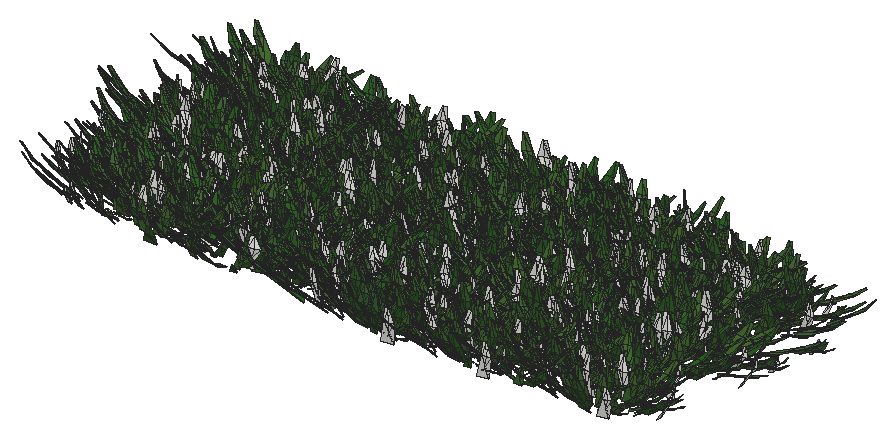
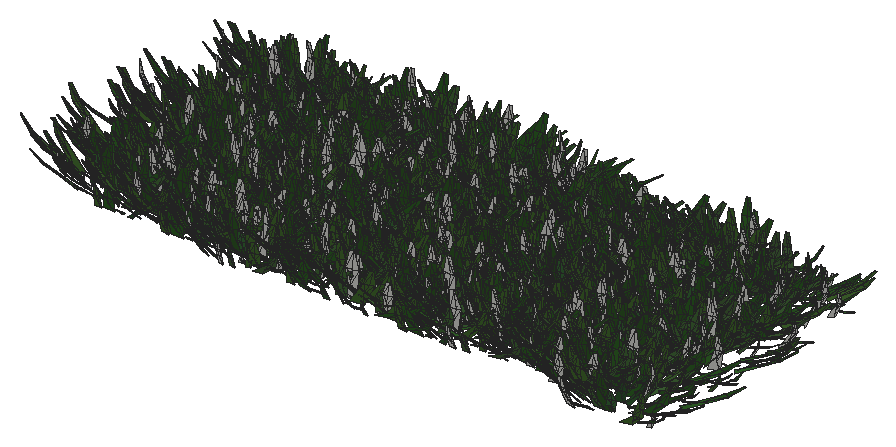
# SketchUp Ruby script. Lengths in inches.
U = 1.inch
M = Sketchup.active_model
def pt(a) = Geom::Point3d.new(a.map { |v| v * U })
def face(e, loops, mat)
  f = e.add_face(loops[0].map { |a| pt(a) })
  loops[1..].each { |l| e.add_face(l.map { |a| pt(a) }).erase! }
  f.material = f.back_material = mat if mat
  f
end
# faces: each face lists its corners as indices into pts; further lists are holes
def faces(e, pts, list, mat = nil) = list.each { |f| face(e, (f[0].is_a?(Array) ? f : [f]).map { |l| l.map { |i| pts[i] } }, mat) }
# xy, xz, yz: faces in a plane at the given z, y or x. An outline is a flat list of corners, or four numbers for a rectangle; further outlines are holes
def ring(l) = l.size == 4 ? [[l[0], l[1]], [l[2], l[1]], [l[2], l[3]], [l[0], l[3]]] : l.each_slice(2).to_a
def flat(e, list, mat, &to3) = list.each { |f| face(e, (f[0].is_a?(Array) ? f : [f]).map { |l| ring(l).map { |u, v| to3.(u, v) } }, mat) }
def xy(e, z, list, mat = nil) = flat(e, list, mat) { |x, y| [x, y, z] }
def xz(e, y, list, mat = nil) = flat(e, list, mat) { |x, z| [x, y, z] }
def yz(e, x, list, mat = nil) = flat(e, list, mat) { |y, z| [x, y, z] }
def lines(e, pts, list) = list.each { |a, b| e.add_line(pt(pts[a]), pt(pts[b])) }
# prism: a flat outline (further loops are holes) pulled along v
def prism(e, loops, v, mat = nil)
  f = face(e, loops, mat); d = Geom::Vector3d.new(v.map { |x| x * U })
  f.pushpull(f.normal.samedirection?(d) ? d.length : -d.length)
end
def box(e, o, s, mat = nil) = prism(e, [[o, [o[0] + s[0], o[1], o[2]], [o[0] + s[0], o[1] + s[1], o[2]], [o[0], o[1] + s[1], o[2]]]], [0, 0, s[2]], mat)
def at(x, y, z, deg = 0) = Geom::Transformation.translation(pt([x, y, z])) * Geom::Transformation.rotation(ORIGIN, Z_AXIS, deg.degrees)
def axes(o, x, y, z) = Geom::Transformation.new([*x, 0, *y, 0, *z, 0, *pt(o).to_a, 1])
def part(name) = M.definitions.add(name)
# library, detail: a bought-in or finely detailed component or shape, given as its bounding box
def library(name, o, s) = part(name).tap { |d| box(d.entities, o, s) }
def detail(e, o, s) = box(e.add_group.entities, o, s)
def put(e, d, t, mat = nil) = e.add_instance(d, t).tap { |i| i.material = mat if mat }
def group(e, t, mat = nil) = e.add_group.tap { |g| g.transformation = t; g.material = mat if mat }.entities
root = M.entities
M.materials.add("Material82").color = [68, 110, 58]
M.materials.add("Material83").color = [48, 90, 38]
M.materials.add("Material84").color = [68, 110, 48]
M.materials.add("Material85").color = [48, 90, 48]
M.materials.add("Material86").color = [58, 110, 58]
M.materials.add("Material87").color = [58, 90, 38]
M.materials.add("Material88").color = [68, 100, 58]
M.materials.add("Material89").color = [48, 100, 38]
c1 = part("grass00")
p = [[-0.6875,0.15,0],[-0.56,0.08,5.52],[-0.04,0.03,2.76],[0.48,-0.02,0],[0.35,-0.02,5.52],[-0.1,-0.14,5.52],
  [-0.12,0.65,8.37],[-0.42,0.65,8.37]]
faces(c1.entities,p,[[0,1,2,3],[3,2,4],[1,5,2],[5,4,2],[1,6,5],[4,5,6],[7,6,1]])
c2 = part("Group16\#1")
put(c2.entities,c1,axes([1.44,-0.61,-0.01],[0.05352,0.12609,0],[-0.10704,0.04543,0.07239],[0.06664,-0.02828,0.11628]),"Material85")
put(c2.entities,c1,axes([0.76,-0.15,-0.01],[0.04676,0.24062,0],[-0.23162,0.04501,0.06642],[0.0652,-0.01267,0.23595]),"Material82")
put(c2.entities,c1,axes([0.79,0.01,-0.01],[-0.00606,0.34651,0],[-0.34381,-0.00602,0.0432],[0.04319,0.00076,0.34386]))
put(c2.entities,c1,axes([1,0.23,-0.01],[-0.07192,0.31144,0],[-0.28722,-0.06632,0.1236],[0.12043,0.02781,0.29478]),"Material84")
put(c2.entities,c1,axes([1.66,0.77,-0.01],[-0.13828,0.29651,0],[-0.21551,-0.1005,0.22471],[0.20365,0.09498,0.23779]),"Material89")
put(c2.entities,c1,axes([0.6875,0.52,-0.01],[-0.18126,0.24051,0],[-0.22746,-0.17142,0.09788],[0.07817,0.05891,0.28481]),"Material84")
put(c2.entities,c1,axes([0.68,0.78,-0.01],[-0.215,0.18688,0],[-0.12385,-0.14248,0.21334],[0.13995,0.16101,0.18878]),"Material82")
put(c2.entities,c1,axes([0.56,1,-0.01],[-0.13756,0.07624,0],[-0.06159,-0.11112,0.0927],[0.04494,0.08108,0.12705]),"Material84")
put(c2.entities,c1,axes([0.2,0.64,-0.01],[-0.23729,0.07254,0],[-0.05711,-0.18681,0.153],[0.04473,0.14632,0.19535]),"Material89")
put(c2.entities,c1,axes([0.0625,0.72,-0.01],[-0.28874,0.02525,0],[-0.02179,-0.24916,0.14647],[0.01276,0.14591,0.25012]),"Material82")
put(c2.entities,c1,axes([-0.08,0.62,-0.01],[-0.34089,-0.04187,0],[0.03255,-0.26504,0.216],[-0.02633,0.21439,0.26703]),"Material89")
put(c2.entities,c1,axes([-0.34,0.98,-0.01],[-0.14314,-0.0493,0],[0.04397,-0.12769,0.06843],[-0.02228,0.0647,0.13505]),"Material89")
put(c2.entities,c1,axes([-0.87,1.45,-0.01],[-0.23488,-0.14114,0],[0.13761,-0.22901,0.06087],[-0.03135,0.05217,0.26717]))
put(c2.entities,c1,axes([-0.72,0.77,-0.01],[-0.14208,-0.13251,0],[0.07209,-0.0773,0.16301],[-0.11118,0.11922,0.1057]),"Material89")
put(c2.entities,c1,axes([-0.62,0.43,-0.01],[-0.14845,-0.21203,0],[0.18654,-0.13061,0.12304],[-0.10079,0.07057,0.22772]),"Material82")
put(c2.entities,c1,axes([-0.68,0.29,-0.01],[-0.13639,-0.32136,0],[0.31723,-0.13464,0.05579],[-0.05136,0.0218,0.34462]),"Material83")
put(c2.entities,c1,axes([-0.64,0.125,-0.01],[-0.0458,-0.23569,0],[0.22124,-0.043,0.08276],[-0.08124,0.01579,0.22538]),"Material86")
put(c2.entities,c1,axes([-1.6,-0.03,-0.01],[0.00576,-0.32897,0],[0.27526,0.00482,0.18018],[-0.18015,-0.00315,0.2753]),"Material84")
put(c2.entities,c1,axes([-1.36,-0.31,-0.01],[0.05718,-0.24765,0],[0.18172,0.04196,0.17267],[-0.16825,-0.03885,0.1865]),"Material89")
put(c2.entities,c1,axes([-1.54,-0.72,-0.01],[0.06537,-0.14017,0],[0.13555,0.06321,0.03939],[-0.0357,-0.01665,0.14956]))
put(c2.entities,c1,axes([-1.19,-0.9,-0.01],[0.09597,-0.12735,0],[0.11214,0.08451,0.07557],[-0.06035,-0.04548,0.14042]),"Material88")
put(c2.entities,c1,axes([-0.47,-0.54,-0.01],[0.11588,-0.10072,0],[0.0618,0.0711,0.12124],[-0.07953,-0.0915,0.0942]))
put(c2.entities,c1,axes([-0.47,-0.84,-0.01],[0.11927,-0.0661,0],[0.06603,0.11913,0.00646],[-0.00313,-0.00565,0.13621]),"Material84")
put(c2.entities,c1,axes([-0.38,-1.24,-0.01],[0.28037,-0.08571,0],[0.0618,0.20215,0.20315],[-0.05939,-0.19428,0.21139]),"Material88")
put(c2.entities,c1,axes([-0.06,-0.66,-0.01],[0.22719,-0.01987,0],[0.01247,0.14255,0.17758],[-0.01547,-0.17691,0.1431]),"Material87")
put(c2.entities,c1,axes([0.11,-0.89,-0.01],[0.14882,0.01828,0],[-0.01058,0.08611,0.12229],[0.01491,-0.12138,0.08676]),"Material85")
put(c2.entities,c1,axes([0.25,-0.72,-0.01],[0.20481,0.07053,0],[-0.06206,0.18022,0.10291],[0.03351,-0.0973,0.1906]),"Material85")
put(c2.entities,c1,axes([0.85,-1.42,-0.01],[0.16481,0.09904,0],[-0.09472,0.15762,0.05616],[0.02893,-0.04814,0.18389]),"Material84")
put(c2.entities,c1,axes([1.01,-1.09,-0.01],[0.21858,0.20385,0],[-0.17495,0.1876,0.15339],[0.10462,-0.11218,0.25652]),"Material89")
put(c2.entities,c1,axes([1.01,-0.71,-0.01],[0.08733,0.12473,0],[-0.06445,0.04512,0.13037],[0.1068,-0.07477,0.07867]),"Material85")
c3 = part("Group15\#1")
put(c3.entities,c2,at(0,0,0))
c4 = part("3darcstudiotree_grass00\#1")
put(c4.entities,c3,at(0,0,0))
put(root,c4,axes([1732.89,309.77,-34.17],[-4.54038,0.15264,0],[-0.30495,-1.41082,-0.04632],[-0.02774,-0.12834,1.89764]))
put(root,c4,axes([1743.27,310.17,-34.17],[-4.30049,-0.14117,0],[0.33609,-1.59238,-0.036],[0.01919,-0.09092,1.9513]))
put(root,c4,axes([1747.83,311.06,-34.17],[4.38861,-0.21228,0],[0.43057,1.38444,-0.03723],[0.02239,0.072,1.30959]))
put(root,c4,axes([1733.82,310.76,-34.17],[-4.13743,-0.67569,0],[1.3247,-1.26157,-0.00358],[0.00873,-0.00832,1.65637]))
put(root,c4,axes([1756.74,310.87,-34.17],[-4.01536,-0.24387,0],[0.54359,-1.39202,-0.03709],[0.03558,-0.0911,1.68681]))
put(root,c4,axes([1737.71,311.1,-34.17],[-2.56412,-1.04956,0],[2.92241,-1.11041,-0.03217],[0.12075,-0.04588,1.58546]))
put(root,c4,axes([1715.12,311.63,-34.17],[2.70248,-1.34249,0],[3.67105,1.14936,-0.06314],[0.18316,0.05735,1.30132]))
put(root,c4,axes([1705.4375,311.57,-34.17],[-0.72323,-1.62263,0],[3.80365,-0.26368,-0.04893],[0.28769,-0.01994,1.72817]))
put(root,c4,axes([1712.21,311.85,-34.17],[3.75674,0.29184,0],[-0.86575,1.73332,-0.03192],[-0.02673,0.05352,1.45488]))
put(root,c4,axes([1758.97,311.9,-34.17],[-1.60231,-1.37282,0],[3.29691,-0.59848,-0.04546],[0.27162,-0.04931,1.78943]))
put(root,c4,axes([1698.92,312.09,-34.17],[2.778,0.72584,0],[-2.53603,1.50959,-0.00365],[-0.00789,0.0047,1.34685]))
put(root,c4,axes([1745.23,312.09,-34.17],[-2.06199,-1.44492,0],[3.43124,-0.76156,-0.05229],[0.2544,-0.05646,1.64764]))
put(root,c4,axes([1722.1,312.32,-34.17],[3.70563,0.39578,0],[-0.96164,1.40032,-0.0432],[-0.06214,0.09049,1.51727]))
put(root,c4,axes([1729.0625,311.99,-34.17],[-2.71187,1.03836,0],[-2.98144,-1.21104,-0.01854],[-0.0717,-0.02913,1.78092]))
put(root,c4,axes([1721.53,313.2,-34.17],[3.3945,-0.58791,0],[1.6844,1.5126,-0.00525],[0.01109,0.00996,1.64886]))
put(root,c4,axes([1700.63,312.94,-34.17],[3.42042,0.9713,0],[-2.12433,1.16348,-0.02682],[-0.10129,0.05548,1.76121]))
put(root,c4,axes([1739.32,313.4,-34.17],[-1.338,-1.30891,0],[3.60545,-0.57321,-0.00075],[0.00363,-0.00058,1.52674]))
put(root,c4,axes([1731.63,313.55,-34.17],[-3.93883,-1.01936,0],[1.86002,-1.11781,-0.04657],[0.18505,-0.11121,1.84036]))
put(root,c4,axes([1759.33,314.01,-34.17],[0.96155,-1.39333,0],[3.31195,0.35548,-0.01758],[0.11319,0.01215,1.71636]))
put(root,c4,axes([1754.3,313.53,-34.17],[-0.63419,1.43243,0],[-3.71512,-0.25582,-0.03794],[-0.18856,-0.01298,1.42617]))
put(root,c4,axes([1727.58,314.07,-34.17],[-2.9141,-1.11595,0],[2.66035,-1.08046,-0.03796],[0.14613,-0.05935,1.58175]))
put(root,c4,axes([1749.7,314.11,-34.17],[-2.17802,-1.23467,0],[3.55396,-0.97507,-0.03629],[0.13271,-0.03641,1.44541]))
put(root,c4,axes([1706.46,314.21,-34.17],[-2.20792,-1.57829,0],[3.78019,-0.82247,-0.0117],[0.05427,-0.01181,1.7149]))
put(root,c4,axes([1714.55,314.45,-34.17],[0.29138,-1.80133,0],[3.99838,0.10059,-0.05413],[0.25015,0.00629,1.39055]))
put(root,c4,axes([1709.8,314.54,-34.17],[4.00255,0.79486,0],[-1.95042,1.52752,-0.03278],[-0.08544,0.06692,1.8841]))
put(root,c4,axes([1743.07,314.43,-34.17],[-3.86108,-0.00922,0],[0.0279,-1.817,-0.0591],[0.00158,-0.1028,1.52309]))
put(root,c4,axes([1734.32,315.13,-34.17],[-1.35898,-1.3893,0],[3.82798,-0.58237,-0.03571],[0.20852,-0.03172,1.92492]))
put(root,c4,axes([1744.05,315.64,-34.17],[-0.67683,-1.69031,0],[4.16932,-0.25965,-0.01303],[0.08012,-0.00499,1.96953]))
put(root,c4,axes([1739.33,315.19,-34.17],[-3.01219,1.1686,0],[-2.47695,-0.99299,-0.0233],[-0.1132,-0.04538,1.83382]))
put(root,c4,axes([1704.75,315.52,-34.17],[3.87339,1.05779,0],[-2.14052,1.21905,-0.05103],[-0.17397,0.09908,1.6877]))
put(root,c4,axes([1712.22,315.8125,-34.17],[-3.28835,-0.7389,0],[1.7462,-1.20864,-0.01205],[0.03007,-0.02081,1.33255]))
put(root,c4,axes([1720.8,316.1,-34.17],[3.72756,0.95688,0],[-1.9535,1.18357,-0.02904],[-0.10466,0.06341,1.7729]))
put(root,c4,axes([1726.33,316.64,-34.17],[2.31636,-1.46039,0],[3.68995,0.91026,-0.01393],[0.05236,0.01292,1.44657]))
put(root,c4,axes([1715.35,316.43,-34.17],[4.20535,0.69684,0],[-1.48182,1.39084,-0.00848],[-0.02193,0.02058,1.91304]))
put(root,c4,axes([1757.0625,316.58,-34.17],[3.11027,0.45791,0],[-1.48719,1.57105,-0.03179],[-0.06172,0.0652,1.76952]))
put(root,c4,axes([1700.06,316.37,-34.17],[-3.34476,-0.15722,0],[0.48645,-1.60959,-0.01308],[0.00826,-0.02735,1.64432]))
put(root,c4,axes([1749.7,316.43,-34.17],[-1.50877,1.48911,0],[-3.61563,-0.56976,-0.0529],[-0.26655,-0.042,1.58349]))
put(root,c4,axes([1727.1,317.29,-34.17],[1.60686,-1.51832,0],[3.56667,0.58707,-0.05171],[0.27066,0.04455,1.64301]))
put(root,c4,axes([1715.09,317.89,-34.17],[3.97377,-0.0043,0],[0.0116,1.66593,-0.02008],[0.00028,0.04042,1.61638]))
put(root,c4,axes([1706,317.88,-34.17],[-0.75362,-1.53541,0],[3.24661,-0.24784,-0.00678],[0.04146,-0.00316,1.54322]))
put(root,c4,axes([1732.9,317.61,-34.17],[-1.22945,1.37189,0],[-3.12548,-0.43563,-0.03966],[-0.20868,-0.02909,1.38647]))
put(root,c4,axes([1745.28,317.54,-34.17],[-2.26778,1.36387,0],[-3.7802,-0.97758,-0.05216],[-0.16857,-0.04359,1.30947]))
put(root,c4,axes([1749.21,318.68,-34.17],[3.45505,-0.2676,0],[0.73895,1.48387,-0.00241],[0.00289,0.0058,1.79003]))
put(root,c4,axes([1753.85,318.27,-34.17],[-3.53984,-0.54558,0],[1.35048,-1.36277,-0.02269],[0.0488,-0.04924,1.64292]))
put(root,c4,axes([1712.36,318.51,-34.17],[2.55644,1.08061,0],[-3.46336,1.27432,-0.03325],[-0.10953,0.0403,1.59934]))
put(root,c4,axes([1739.08,318.18,-34.17],[-0.71352,1.56405,0],[-4.14814,-0.29432,-0.02584],[-0.10481,-0.00744,1.30174]))
put(root,c4,axes([1698.32,318.26,-34.17],[-0.26231,1.84263,0],[-3.30675,-0.07321,-0.00552],[-0.03272,-0.00072,1.47331]))
put(root,c4,axes([1720.77,318.43,-34.17],[0.91997,1.29984,0],[-3.25818,0.35865,-0.02635],[-0.1448,0.01594,1.4463]))
put(root,c4,axes([1721.68,319.7,-34.17],[3.30024,-0.68967,0],[2.06464,1.53659,-0.00115],[0.00232,0.00173,1.42878]))
put(root,c4,axes([1731.24,320.24,-34.17],[2.55399,-1.11237,0],[2.83561,1.01258,-0.04299],[0.17745,0.06336,1.59659]))
put(root,c4,axes([1700.1875,320.08,-34.17],[3.21897,1.19921,0],[-3.23164,1.34914,-0.01632],[-0.04651,0.01942,1.46423]))
put(root,c4,axes([1712.57,319.8,-34.17],[-0.44896,1.44211,0],[-4.03082,-0.19517,-0.03564],[-0.19872,-0.00962,1.71014]))
put(root,c4,axes([1745.27,319.67,-34.17],[-1.84352,1.61201,0],[-4.26993,-0.75947,-0.03185],[-0.15055,-0.02678,1.82087]))
put(root,c4,axes([1729.17,319.98,-34.17],[-3.29654,-0.72222,0],[2.17338,-1.54289,-0.02959],[0.0707,-0.05019,1.65043]))
put(root,c4,axes([1704.93,320.74,-34.17],[1.85229,-1.14191,0],[3.43107,0.86561,-0.02581],[0.11483,0.02897,1.61243]))
put(root,c4,axes([1714.76,320.76,-34.17],[0.37581,-1.33084,0],[4.05324,0.17801,-0.00391],[0.01773,0.00078,1.39627]))
put(root,c4,axes([1738.8,321.01,-34.17],[3.4977,-1.17788,0],[2.34178,1.08154,-0.01134],[0.04108,0.01897,1.5074]))
put(root,c4,axes([1749.75,320.44,-34.17],[-2.729,0.78907,0],[-2.0311,-1.09252,-0.03589],[-0.15909,-0.08558,1.93035]))
put(root,c4,axes([1755.65,320.46,-34.17],[-2.28466,1.61729,0],[-3.8326,-0.84205,-0.0557],[-0.22938,-0.0504,1.55009]))
put(root,c4,axes([1757.05,321.7,-34.17],[1.96831,-1.06776,0],[3.09361,0.88694,-0.02782],[0.14847,0.04257,1.89124]))
put(root,c4,axes([1742.85,321.65,-34.17],[0.83797,-1.39271,0],[3.20742,0.30015,-0.04624],[0.35526,0.03324,1.95114]))
put(root,c4,axes([1740.82,321.81,-34.17],[3.50844,-0.55754,0],[1.25662,1.22985,-0.02314],[0.04614,0.04516,1.34449]))
put(root,c4,axes([1697.96,321.85,-34.17],[3.19452,-0.59612,0],[1.46474,1.2208,-0.01286],[0.03129,0.02608,1.45976]))
put(root,c4,axes([1759.83,321.67,-34.17],[-1.71956,-1.37213,0],[4.12265,-0.80354,-0.04891],[0.23955,-0.04669,1.88309]))
put(root,c4,axes([1704.26,321.92,-34.17],[0.90068,-1.41561,0],[4.53027,0.44829,-0.03647],[0.13709,0.01357,1.35653]))
put(root,c4,axes([1709.53,321.66,-34.17],[-2.78639,1.08314,0],[-3.04744,-1.21928,-0.00446],[-0.01393,-0.00557,1.44777]))
put(root,c4,axes([1721.67,322.33,-34.17],[-2.22834,-1.37792,0],[3.47538,-0.87412,-0.04256],[0.18098,-0.04552,1.55835]))
put(root,c4,axes([1748.92,322.67,-34.17],[-3.88555,-0.79581,0],[2.02489,-1.53765,-0.03725],[0.08107,-0.06156,1.55507]))
put(root,c4,axes([1729.59,322.68,-34.17],[-4.41332,-0.66754,0],[1.63018,-1.67623,-0.02874],[0.04038,-0.04152,1.33872]))
put(root,c4,axes([1718.25,322.74,-34.17],[-3.79387,-0.48377,0],[1.38418,-1.6883,-0.04655],[0.0671,-0.08184,1.58019]))
put(root,c4,axes([1732.08,322.64,-34.17],[-4.27576,-0.00967,0],[0.01971,-1.35519,-0.00073],[0.00002,-0.00168,1.50826]))
put(root,c4,axes([1740.23,324.16,-34.17],[1.98892,-1.13086,0],[3.89758,1.06614,-0.02169],[0.07891,0.02158,1.57389]))
put(root,c4,axes([1716.92,324.52,-34.17],[2.33801,-1.27151,0],[3.45385,0.98774,-0.00976],[0.0468,0.01338,1.89325]))
put(root,c4,axes([1756.93,324.23,-34.17],[-3.20918,-1.37059,0],[3.45166,-1.25697,-0.04946],[0.15315,-0.05577,1.48426]))
put(root,c4,axes([1710.22,324.53,-34.17],[3.64852,0.24315,0],[-0.61045,1.42466,-0.04218],[-0.04748,0.11082,1.85529]))
put(root,c4,axes([1700.63,324.15,-34.17],[-2.66899,1.32243,0],[-3.00544,-0.94339,-0.02078],[-0.10429,-0.03273,1.84714]))
put(root,c4,axes([1704.52,324.96,-34.17],[4.17155,-0.17702,0],[0.50263,1.84221,-0.03237],[0.01504,0.05512,1.52951]))
put(root,c4,axes([1743.8,324.84,-34.17],[2.88531,0.9286,0],[-2.55752,1.23593,-0.03119],[-0.12387,0.05986,1.90467]))
put(root,c4,axes([1731.4375,324.58,-34.17],[-2.10798,1.40451,0],[-3.51427,-0.82033,-0.03668],[-0.20421,-0.04767,1.98009]))
put(root,c4,axes([1727.58,324.83,-34.17],[1.47468,1.38827,0],[-3.83437,0.63347,-0.03717],[-0.17802,0.02941,1.61797]))
put(root,c4,axes([1759.41,324.8,-34.17],[0.13535,1.36053,0],[-4.14262,0.0641,-0.00595],[-0.03791,0.00059,1.98232]))
put(root,c4,axes([1720.42,324.7,-34.17],[-3.1837,0.9292,0],[-2.49148,-1.32767,-0.01624],[-0.05606,-0.02987,1.82169]))
put(root,c4,axes([1750.54,325.44,-34.17],[-4.08688,-0.61044,0],[1.62889,-1.6961,-0.00084],[0.00115,-0.0012,1.34285]))
put(root,c4,axes([1743.04,326.12,-34.17],[1.67099,-1.73753,0],[3.10475,0.46439,-0.00605],[0.0444,0.00664,1.95327]))
put(root,c4,axes([1699.73,326.34,-34.17],[4.2125,0.29861,0],[-0.756,1.65872,-0.00017],[-0.00017,0.00037,1.78268]))
put(root,c4,axes([1727.35,326.29,-34.17],[4.05845,0.38101,0],[-1.01694,1.68476,-0.06215],[-0.0714,0.11828,1.63292]))
put(root,c4,axes([1754.44,326.37,-34.17],[-1.7024,-1.44396,0],[3.0538,-0.55996,-0.04244],[0.29035,-0.05324,1.90455]))
put(root,c4,axes([1717.25,326.42,-34.17],[-0.84806,-1.31842,0],[3.86352,-0.38651,-0.05601],[0.32758,-0.03277,1.80254]))
put(root,c4,axes([1712.34,326.47,-34.17],[-2.64127,-0.90818,0],[2.55598,-1.15614,-0.03875],[0.14904,-0.06742,1.70607]))
put(root,c4,axes([1732.28,326.41,-34.17],[-3.43779,0.5694,0],[-1.45981,-1.37078,-0.01995],[-0.04437,-0.04166,1.62326]))
put(root,c4,axes([1707.22,326.62,-34.17],[-2.26233,1.10327,0],[-2.6855,-0.85647,-0.00747],[-0.03039,-0.00969,1.35493]))
put(root,c4,axes([1760.52,326.58,-34.17],[-3.44248,1.19972,0],[-2.84327,-1.26888,-0.04086],[-0.12277,-0.05479,1.46035]))
put(root,c4,axes([1737.26,327.37,-34.17],[3.38923,-0.39007,0],[1.26949,1.71555,-0.04654],[0.05157,0.06969,1.34343]))
put(root,c4,axes([1721.23,327.55,-34.17],[-1.79663,-1.22383,0],[3.52148,-0.80403,-0.02105],[0.11606,-0.0265,1.94345]))
put(root,c4,axes([1751.6875,327.4375,-34.17],[-4.21718,-0.04667,0],[0.09647,-1.35575,-0.03959],[0.00846,-0.11883,1.96257]))
put(root,c4,axes([1710.93,328.35,-34.17],[-3.15245,-0.45856,0],[1.56973,-1.67838,-0.02933],[0.05139,-0.05494,1.72129]))
put(root,c4,axes([1747.87,328.42,-34.17],[1.70731,1.1244,0],[-2.88773,0.68196,-0.04808],[-0.30467,0.07195,1.86326]))
put(root,c4,axes([1754.88,328.375,-34.17],[-2.99752,0.92431,0],[-2.30263,-1.1614,-0.02144],[-0.09164,-0.04622,1.94421]))
put(root,c4,axes([1726.02,328.69,-34.17],[-0.05283,1.30539,0],[-4.56112,-0.02871,-0.04794],[-0.23084,-0.00145,1.64652]))
put(root,c4,axes([1700.16,328.75,-34.17],[-4.04939,0.05434,0],[-0.15117,-1.75202,-0.01213],[-0.00231,-0.02678,1.86653]))
put(root,c4,axes([1745.98,329.47,-34.17],[3.97524,-0.29729,0],[0.87691,1.8237,-0.05959],[0.04913,0.10217,1.56123]))
put(root,c4,axes([1717.47,329.22,-34.17],[4.25696,0.81021,0],[-1.71809,1.40397,-0.05424],[-0.1086,0.08874,1.36476]))
put(root,c4,axes([1721.2,328.85,-34.17],[-2.04292,1.4828,0],[-3.7482,-0.80316,-0.0267],[-0.09668,-0.02072,1.31753]))
put(root,c4,axes([1731.3,329.62,-34.17],[3.62862,0.35052,0],[-1.11939,1.8023,-0.01455],[-0.01942,0.03128,1.97892]))
put(root,c4,axes([1705.63,329.82,-34.17],[2.6006,-1.2072,0],[3.21281,1.07644,-0.02612],[0.11842,0.03968,1.8801]))
put(root,c4,axes([1737.32,329.65,-34.17],[-3.56945,0.98002,0],[-2.54129,-1.43957,-0.02528],[-0.0766,-0.04339,1.76765]))
put(root,c4,axes([1721.78,330.68,-34.17],[0.7854,-1.46662,0],[3.6757,0.30614,-0.00249],[0.01359,0.00113,1.57305]))
put(root,c4,axes([1740.74,330.8125,-34.17],[1.68218,-1.47179,0],[3.03421,0.53937,-0.02223],[0.13236,0.02353,1.62899]))
put(root,c4,axes([1749.18,330.9375,-34.17],[0.3333,-1.68825,0],[3.84573,0.11808,-0.01871],[0.11577,0.00355,1.79426]))
put(root,c4,axes([1711.37,330.71,-34.17],[3.57061,0.64267,0],[-1.40632,1.21522,-0.03533],[-0.10777,0.09312,1.86502]))
put(root,c4,axes([1698.97,330.5625,-34.17],[-2.58541,-0.85496,0],[2.80483,-1.31917,-0.0116],[0.03194,-0.01502,1.40225]))
put(root,c4,axes([1756.55,331.1,-34.17],[3.17331,-0.50017,0],[1.66687,1.64477,-0.02256],[0.03879,0.03827,1.55958]))
put(root,c4,axes([1716.875,330.6,-34.17],[-3.33443,-0.23634,0],[0.70723,-1.55188,-0.01818],[0.01451,-0.03184,1.35222]))
put(root,c4,axes([1728.25,331.65,-34.17],[-1.63027,-1.73131,0],[4.11958,-0.60332,-0.00006],[0.00033,-0.00005,1.81412]))
put(root,c4,axes([1742.84,331.4,-34.17],[-2.03219,1.40442,0],[-2.95743,-0.66557,-0.04437],[-0.22116,-0.04977,1.46464]))
put(root,c4,axes([1707.35,331.75,-34.17],[0.61227,1.37165,0],[-4.42146,0.30696,-0.06022],[-0.31422,0.02181,1.78296]))
put(root,c4,axes([1761.31,331.56,-34.17],[-3.77371,1.09403,0],[-2.05317,-1.10148,-0.00523],[-0.01755,-0.00942,1.47184]))
put(root,c4,axes([1733.24,331.97,-34.17],[1.42302,1.52353,0],[-4.19442,0.60932,-0.04046],[-0.17686,0.02569,1.56076]))
put(root,c4,axes([1735.23,332.93,-34.17],[3.4755,-0.56156,0],[1.30477,1.25594,-0.00746],[0.01674,0.01612,1.52751]))
put(root,c4,axes([1710.99,332.83,-34.17],[-1.74555,-1.44076,0],[3.95857,-0.74592,-0.00689],[0.03295,-0.00621,1.74288]))
put(root,c4,axes([1751.85,332.7,-34.17],[-0.75802,1.26839,0],[-3.28645,-0.30547,-0.04738],[-0.26314,-0.02446,1.4441]))
put(root,c4,axes([1740,333.17,-34.17],[-1.97999,-1.67359,0],[3.87039,-0.71217,-0.01753],[0.07436,-0.01368,1.49864]))
put(root,c4,axes([1746.11,332.85,-34.17],[0.81482,1.77329,0],[-4.44159,0.31742,-0.02342],[-0.11628,0.00831,1.70718]))
put(root,c4,axes([1726.61,332.92,-34.17],[0.46872,1.37145,0],[-4.27579,0.22728,-0.05207],[-0.28533,0.01517,1.7882]))
put(root,c4,axes([1758.85,332.8,-34.17],[-1.06746,1.42925,0],[-3.87706,-0.45036,-0.01201],[-0.05554,-0.00645,1.46096]))
put(root,c4,axes([1720.44,333.8,-34.17],[3.33835,-0.04276,0],[0.15045,1.82678,-0.05593],[0.00839,0.10182,1.60461]))
put(root,c4,axes([1755.14,333.75,-34.17],[-0.95803,-1.53129,0],[3.44538,-0.33525,-0.01268],[0.07432,-0.00723,1.60602]))
put(root,c4,axes([1715.06,333.9,-34.17],[0.3233,-1.61244,0],[3.70268,0.11546,-0.00365],[0.02017,0.00063,1.54435]))
put(root,c4,axes([1705.17,333.31,-34.17],[-3.72731,0.81099,0],[-1.84954,-1.32207,-0.01481],[-0.0358,-0.02559,1.43556]))
put(root,c4,axes([1701.88,333.43,-34.17],[-1.62678,1.3546,0],[-3.70168,-0.6914,-0.05633],[-0.31213,-0.0583,1.88219]))
put(root,c4,axes([1755.67,335.17,-34.17],[0.20206,-1.72347,0],[4.27325,0.07792,-0.04434],[0.21389,0.0039,1.54852]))
put(root,c4,axes([1704.15,335.47,-34.17],[1.41685,-1.43454,0],[3.76136,0.57778,-0.0174],[0.0698,0.01072,1.30214]))
put(root,c4,axes([1700.66,334.875,-34.17],[-3.91283,-0.66077,0],[1.78522,-1.64415,-0.00601],[0.01088,-0.01002,1.5624]))
put(root,c4,axes([1760.07,335.08,-34.17],[-3.8816,-0.56323,0],[1.5517,-1.6632,-0.01333],[0.02356,-0.02525,1.7245]))
put(root,c4,axes([1736.99,335.43,-34.17],[3.63174,0.64343,0],[-1.49454,1.312,-0.04301],[-0.1083,0.09507,1.6797]))
put(root,c4,axes([1709.31,335.92,-34.17],[-1.36397,-1.5291,0],[3.40561,-0.47247,-0.03242],[0.15123,-0.02098,1.33794]))
put(root,c4,axes([1748.12,335.38,-34.17],[-2.70631,1.45447,0],[-3.636,-1.05223,-0.06171],[-0.25363,-0.0734,1.72322]))
put(root,c4,axes([1732.93,335.71,-34.17],[1.95907,1.41788,0],[-3.34699,0.71925,-0.025],[-0.15312,0.03291,1.99255]))
put(root,c4,axes([1722.26,336.08,-34.17],[-0.62966,-1.28695,0],[4.54348,-0.34574,-0.02161],[0.1197,-0.00911,1.95654]))
put(root,c4,axes([1714.65,335.76,-34.17],[-3.55761,-0.37183,0],[0.9234,-1.37408,-0.01321],[0.02436,-0.03625,1.9444]))
put(root,c4,axes([1744.93,335.77,-34.17],[-1.83042,1.58988,0],[-3.0568,-0.54735,-0.0444],[-0.26156,-0.04683,1.62807]))
put(root,c4,axes([1726.38,336.05,-34.17],[-3.95397,0.70682,0],[-1.69994,-1.479,-0.00714],[-0.01245,-0.01084,1.30481]))
put(root,c4,axes([1709.66,337.1,-34.17],[4.34464,0.20061,0],[-0.52956,1.78372,-0.02723],[-0.01491,0.05022,1.60719]))
put(root,c4,axes([1704.85,337.02,-34.17],[1.20267,1.27774,0],[-3.21983,0.47135,-0.04291],[-0.22552,0.03301,1.44315]))
put(root,c4,axes([1743.14,338.01,-34.17],[1.32812,-1.21732,0],[3.65511,0.62022,-0.02985],[0.14197,0.02409,1.54439]))
put(root,c4,axes([1716.55,337.8,-34.17],[-1.97159,-1.316,0],[4.00038,-0.93213,-0.05519],[0.24758,-0.05769,1.81465]))
put(root,c4,axes([1699.65,337.59,-34.17],[-4.26775,-0.24104,0],[0.59342,-1.63411,-0.00988],[0.00789,-0.02172,1.76639]))
put(root,c4,axes([1750.74,337.4375,-34.17],[-3.54904,1.16368,0],[-2.54993,-1.20953,-0.00935],[-0.03236,-0.01535,1.61847]))
put(root,c4,axes([1737.34,337.55,-34.17],[-3.22115,0.33319,0],[-1.15137,-1.73117,-0.03948],[-0.04657,-0.07003,1.58152]))
put(root,c4,axes([1753.43,337.82,-34.17],[-3.58911,0.17625,0],[-0.41421,-1.31187,-0.03309],[-0.02615,-0.08283,1.60704]))
put(root,c4,axes([1759.39,337.73,-34.17],[-3.46015,1.06405,0],[-2.06953,-1.04669,-0.02241],[-0.08068,-0.04081,1.47722]))
put(root,c4,axes([1721.12,337.8,-34.17],[-3.47223,1.22215,0],[-3.01377,-1.3317,-0.01139],[-0.0395,-0.01745,1.76647]))
put(root,c4,axes([1731.67,337.97,-34.17],[-1.73682,1.47733,0],[-4.1333,-0.75577,-0.04346],[-0.21523,-0.03935,1.86413]))
put(root,c4,axes([1726.4,338.51,-34.17],[-0.9909,1.30306,0],[-3.23471,-0.38257,-0.04553],[-0.22482,-0.02659,1.30482]))
put(root,c4,axes([1742.97,339.13,-34.17],[-1.94812,-1.05267,0],[3.13916,-0.90354,-0.00015],[0.00082,-0.00024,1.94435]))
put(root,c4,axes([1698.93,339.66,-34.17],[2.46062,-1.19689,0],[3.08233,0.98555,-0.02965],[0.1062,0.03396,1.3715]))
